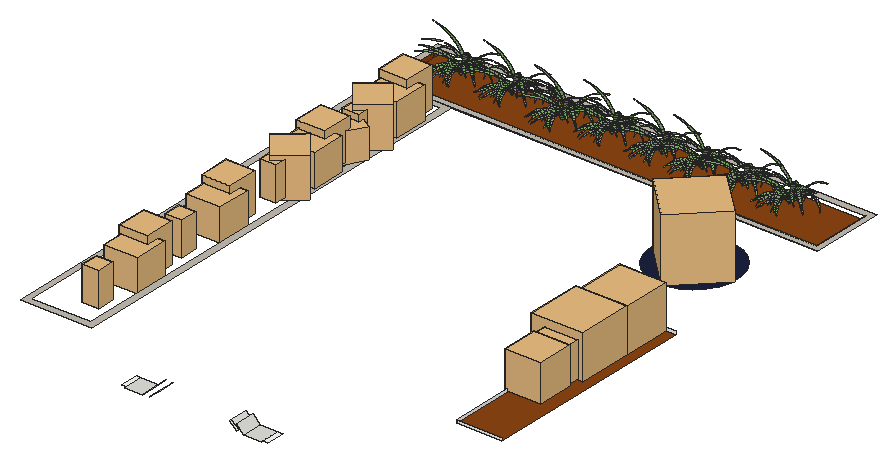
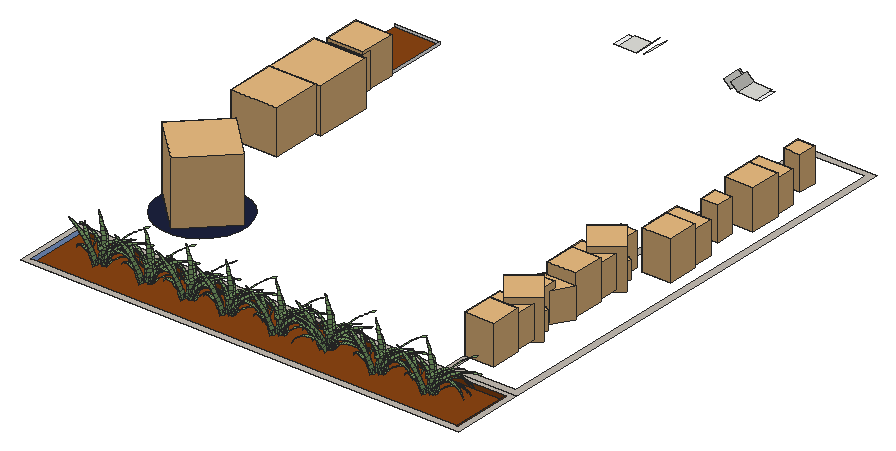
# SketchUp Ruby script. Lengths in inches.
U = 1.inch
M = Sketchup.active_model
def pt(a) = Geom::Point3d.new(a.map { |v| v * U })
def face(e, loops, mat)
  f = e.add_face(loops[0].map { |a| pt(a) })
  loops[1..].each { |l| e.add_face(l.map { |a| pt(a) }).erase! }
  f.material = f.back_material = mat if mat
  f
end
# faces: each face lists its corners as indices into pts; further lists are holes
def faces(e, pts, list, mat = nil) = list.each { |f| face(e, (f[0].is_a?(Array) ? f : [f]).map { |l| l.map { |i| pts[i] } }, mat) }
# xy, xz, yz: faces in a plane at the given z, y or x. An outline is a flat list of corners, or four numbers for a rectangle; further outlines are holes
def ring(l) = l.size == 4 ? [[l[0], l[1]], [l[2], l[1]], [l[2], l[3]], [l[0], l[3]]] : l.each_slice(2).to_a
def flat(e, list, mat, &to3) = list.each { |f| face(e, (f[0].is_a?(Array) ? f : [f]).map { |l| ring(l).map { |u, v| to3.(u, v) } }, mat) }
def xy(e, z, list, mat = nil) = flat(e, list, mat) { |x, y| [x, y, z] }
def xz(e, y, list, mat = nil) = flat(e, list, mat) { |x, z| [x, y, z] }
def yz(e, x, list, mat = nil) = flat(e, list, mat) { |y, z| [x, y, z] }
def lines(e, pts, list) = list.each { |a, b| e.add_line(pt(pts[a]), pt(pts[b])) }
# prism: a flat outline (further loops are holes) pulled along v
def prism(e, loops, v, mat = nil)
  f = face(e, loops, mat); d = Geom::Vector3d.new(v.map { |x| x * U })
  f.pushpull(f.normal.samedirection?(d) ? d.length : -d.length)
end
def box(e, o, s, mat = nil) = prism(e, [[o, [o[0] + s[0], o[1], o[2]], [o[0] + s[0], o[1] + s[1], o[2]], [o[0], o[1] + s[1], o[2]]]], [0, 0, s[2]], mat)
def at(x, y, z, deg = 0) = Geom::Transformation.translation(pt([x, y, z])) * Geom::Transformation.rotation(ORIGIN, Z_AXIS, deg.degrees)
def axes(o, x, y, z) = Geom::Transformation.new([*x, 0, *y, 0, *z, 0, *pt(o).to_a, 1])
def part(name) = M.definitions.add(name)
# library, detail: a bought-in or finely detailed component or shape, given as its bounding box
def library(name, o, s) = part(name).tap { |d| box(d.entities, o, s) }
def detail(e, o, s) = box(e.add_group.entities, o, s)
def put(e, d, t, mat = nil) = e.add_instance(d, t).tap { |i| i.material = mat if mat }
def group(e, t, mat = nil) = e.add_group.tap { |g| g.transformation = t; g.material = mat if mat }.entities
root = M.entities
M.materials.add("[0043_SaddleBrown]").color = [139, 69, 19]
M.materials.add("[0119_RosyBrown]").color = [29, 34, 63]
M.materials.add("[Color L01]").color = [158, 192, 255]
M.materials.add("[Color M00]").color = [255, 255, 255]
M.materials.add("[Field Rectangle Tile]").color = [196, 189, 179]
M.materials.add("dianella").color = [131, 171, 111]
c1 = library("Group38\#2",[14.01,28.44,-23.43],[18.58,18.32,38.89])
c2 = library("Group20\#1",[-20.81,-17.08,3.79],[39.86,39.43,37.51])
c3 = library("Group\#130",[-7.34,-1.2,0],[38.67,35.81,49.04])
c4 = library("Group\#339",[-7.85,-8.32,-6.76],[58.34,57.85,58.74])
c5 = library("Group\#332",[-8.56,-8.18,-3.7],[55.71,56.19,59.24])
c6 = library("Group\#329",[-12.44,-11,-10.61],[94.39,87.27,76.58])
c7 = library("Group\#292",[-21.05,-15.88,-13.81],[107.65,102.98,97.72])
c8 = library("Group\#74",[-84.69,-90.07,-0.36],[176.51,175.13,171.4])
c9 = library("Areca palm plant",[0,0,0],[49.1,36.6,54.46])
c10 = library("Water tank",[0,0,0],[57.22,57.22,62.99])
c11 = part("Shape Bender Component\#4")
p = [[0.27,1.78,0.46],[1.95,1.8,3.35],[1.95,4.67,3.35],[0.27,4.68,0.46],[3.06,1.81,4.8],[3.875,1.84,5.87],
  [3.875,4.64,5.87],[3.06,4.66,4.8],[6,1.9,8],[6,4.58,8],[27.35,3.23,6.09],[25.57,3.4375,7.9],
  [25.57,3.03,7.9],[23.28,2.8,9.61],[23.28,3.67,9.61],[7.08,1.93,8.8],[8.3,1.99,9.69],[8.3,4.5,9.69],
  [7.08,4.55,8.8],[23.04,2.78,9.74],[23.04,3.69,9.74],[20.86,3.86,10.86],[20.86,2.625,10.86],[10.73,2.08,10.92],
  [10.73,4.41,10.92],[12.13,2.13,11.33],[13.24,2.19,11.66],[13.24,4.3,11.66],[12.13,4.36,11.33],[18.35,2.46,11.63],
  [18.35,4.03,11.63],[15.79,2.32,11.89],[17.75,2.42,11.69],[17.75,4.07,11.69],[15.79,4.17,11.89]]
faces(c11.entities,p,[[0,1,2,3],[1,4,5,6,7,2],[5,8,9,6],[10,11,12],[13,12,11,14],[15,16,17,18,9,8],[19,13,14,20,21,22],[16,23,24,17],
  [23,25,26,27,28,24],[29,22,21,30],[31,32,29,30,33,34],[26,31,34,27]],"dianella")
c12 = part("Shape Bender Component\#7")
p = [[0.01,0.94,1.17],[0.04,0.96,6.32],[0.04,4.67,6.32],[0.01,4.68,1.17],[0.42,0.98,10.52],[0.51,1,11.45],
  [0.51,4.64,11.45],[0.42,4.66,10.52],[1.4,1.07,16.52],[1.4,4.57,16.52],[2.48,1.13,20.62],[2.71,1.16,21.49],
  [2.71,4.49,21.49],[2.48,4.52,20.625],[4.4375,1.21,26.32],[4.4375,4.46,26.32],[6.56,1.22,30.98],[6.56,4.47,30.98],
  [9.06,1.29,35.43],[9.06,4.38,35.43],[11.92,1.42,39.64],[11.92,4.23,39.64],[15.13,1.74,43.57],[15.13,4,43.57],
  [18.65,2.08,47.2],[18.65,3.67,47.2],[22.46,2.47,50.5],[22.46,3.14,50.5],[25.84,2.81,52.95]]
faces(c12.entities,p,[[0,1,2,3],[1,4,5,6,7,2],[5,8,9,6],[10,11,12,13,9,8],[11,14,15,12],[14,16,17,15],[16,18,19,17],[18,20,21,19],
  [20,22,23,21],[22,24,25,23],[24,26,27,25],[28,27,26]],"dianella")
c13 = part("Shape Bender Component\#5")
p = [[0.17,0.01,0.72],[1.09,0.03,4.5625],[1.09,3.73,4.5625],[0.17,3.75,0.72],[2.23,0.05,7.59],[2.48,0.0625,8.26],
  [2.48,3.71,8.26],[2.23,3.72,7.59],[4.33,0.14,11.74],[4.33,3.64,11.74],[6.2,0.2,14.41],[6.6,0.22,14.97],
  [6.6,3.56,14.97],[6.2,3.58,14.41],[9.26,0.35,17.88],[9.26,3.43,17.88],[12.27,0.4,20.43],[12.27,3.38,20.43],
  [15.58,0.51,22.59],[15.58,3.27,22.59],[19.13,0.73,24.3],[19.13,3.14,24.3],[22.875,1.08,25.56],[22.875,2.85,25.56],
  [26.75,1.47,26.33],[26.75,2.49,26.33],[30.68,1.86,26.6],[30.68,2.125,26.6],[33.95,1.875,26.45]]
faces(c13.entities,p,[[0,1,2,3],[1,4,5,6,7,2],[5,8,9,6],[8,10,11,12,13,9],[11,14,15,12],[14,16,17,15],[16,18,19,17],[18,20,21,19],
  [20,22,23,21],[22,24,25,23],[24,26,27,25],[28,27,26]],"dianella")
xy(root,281.8125,[[30,509.79,450,570]],"[0043_SaddleBrown]")
xy(root,285.0625,[[172.5,4,190.5,24],[289.5,4,307.5,24]])
xy(root,285.0625,[[168,6,172.5,24],[307.5,6,312,24]],"[Color M00]")
xy(root,286.25,[[398.2,388.3,408.88,390.95,418.5,396.27,426.42,403.9,432.1,413.32,435.14,423.88,435.35,434.88,432.7,445.55,427.38,455.18,419.75,463.1,410.34,468.77,399.77,471.82,388.77,472.02,378.1,469.375,368.47,464.06,360.55,456.43,354.88,447.01,351.83,436.44,351.63,425.45,354.27,414.77,359.59,405.15,367.22,397.23,376.64,391.55,387.21,388.51]],"[0119_RosyBrown]")
xy(root,286.25,[[[24,60.88,94.68,503.79],[30,66.88,88.68,497.79]],[[24,503.79,456,576],[30,509.79,450,570]]],"[Field Rectangle Tile]")
xy(root,289.375,[[411,114.58,456,328.96]],"[0043_SaddleBrown]")
xz(root,114.58,[[411,289.375,456,292.1875]],"[Color M00]")
xz(root,328.96,[[411,289.375,456,292.1875]],"[Color M00]")
xz(root,509.79,[[30,281.8125,94.68,286.25],[94.68,281.8125,350.9,286.25],[350.9,281.8125,410.59,286.25],[410.59,281.8125,450,286.25]],"[0043_SaddleBrown]")
yz(root,30,[[509.79,281.8125,570,286.25]],"[0043_SaddleBrown]")
yz(root,411,[[114.58,289.375,328.96,292.1875]],"[Color M00]")
yz(root,450,[[509.79,281.8125,570,286.25]],"[Color L01]")
p = [[190.5,24,285.0625],[190.5,4,285.0625],[196.91,4,292.04],[196.91,24,292.04],[283.09,24,292.04],[283.09,4,292.04],
  [289.5,4,285.0625],[289.5,24,285.0625],[196.93,6,286.04],[204.32,6,291.98],[204.32,4,291.98],[196.93,4,286.04],
  [275.8,6,291.98],[283.2,6,286.04],[283.2,4,286.04],[275.8,4,291.98],[196.93,24,286.04],[204.32,24,291.98],
  [275.8,24,291.98],[283.2,24,286.04]]
faces(root,p,[[0,1,2,3],[4,5,6,7],[8,9,10,11],[12,13,14,15],[9,8,16,17],[13,12,18,19]])
put(root,c1,axes([46.13,67.14,301.625],[0.8848,0,0],[0,0.94674,0],[0,0,0.85826]))
put(root,c2,axes([69.2,148.27,278.23],[0,0.85,0],[-0.85,0,0],[0,0,0.85]))
put(root,c3,axes([75.17,158.2,281.45],[0,0.79,0],[-0.79,0,0],[0,0,0.79]))
put(root,c4,axes([439.2,181.99,294.74],[0,0.616,0],[-0.616,0,0],[0,0,0.616]))
put(root,c1,axes([46.13,168.95,301.625],[0.8848,0,0],[0,0.94674,0],[0,0,0.85826]))
put(root,c5,axes([436.17,209.26,292.1875],[0,0.58004,0],[-0.58004,0,0],[0,0,0.58004]))
put(root,c2,axes([69.2,250.08,278.23],[0,0.85,0],[-0.85,0,0],[0,0,0.85]))
put(root,c6,axes([439.55,233.71,293.78],[0,0.58004,0],[-0.58004,0,0],[0,0,0.58004]))
put(root,c3,axes([75.17,260.02,281.45],[0,0.79,0],[-0.79,0,0],[0,0,0.79]))
put(root,c1,axes([59.43,268.9,310.82],[0.8848,0,0],[0,0.94674,0],[0,0,0.85826]))
put(root,c7,axes([439.1,290.93,294.59],[0,0.44269,0],[-0.44269,0,0],[0,0,0.44269]))
put(root,c8,axes([78.46,314.11,288.7],[-0.04961,-0.08593,0],[0.08593,-0.04961,0],[0,0,0.10522]))
put(root,c9,axes([57.34,326.66,288.73],[0.45017,-0.56191,0],[0.66137,0.52986,0],[0,0,0.72]))
put(root,c8,axes([78.46,341.36,288.7],[-0.04961,-0.08593,0],[0.08593,-0.04961,0],[0,0,0.10522]))
put(root,c2,axes([82.5,350.03,287.42],[0,0.85,0],[-0.85,0,0],[0,0,0.85]))
put(root,c8,axes([78.46,361.43,288.7],[-0.04961,-0.08593,0],[0.08593,-0.04961,0],[0,0,0.10522]))
put(root,c3,axes([88.47,359.97,290.64],[0,0.79,0],[-0.79,0,0],[0,0,0.79]))
put(root,c8,axes([80.72,391.29,288.72],[-0.08133,-0.14087,0],[0.14087,-0.08133,0],[0,0,0.1725]))
put(root,c1,axes([59.43,370.72,310.82],[0.8848,0,0],[0,0.94674,0],[0,0,0.85826]))
put(root,c8,axes([78.46,415.93,288.7],[-0.04961,-0.08593,0],[0.08593,-0.04961,0],[0,0,0.10522]))
put(root,c9,axes([57.34,428.47,288.73],[0.45017,-0.56191,0],[0.66137,0.52986,0],[0,0,0.72]))
put(root,c10,at(395.83,385.39,286.25,45))
put(root,c8,axes([78.46,443.18,288.7],[-0.04961,-0.08593,0],[0.08593,-0.04961,0],[0,0,0.10522]))
put(root,c2,axes([82.5,451.85,287.42],[0,0.85,0],[-0.85,0,0],[0,0,0.85]))
put(root,c8,axes([78.46,463.24,288.7],[-0.04961,-0.08593,0],[0.08593,-0.04961,0],[0,0,0.10522]))
put(root,c3,axes([88.47,461.78,290.64],[0,0.79,0],[-0.79,0,0],[0,0,0.79]))
put(root,c11,axes([179.97,534.78,303.24],[0.24384,-0.52892,-0.4943],[-0.96778,-0.07931,-0.14256],[-0.0628,-0.83154,0.27772]))
put(root,c11,axes([181.1,538.37,290.98],[0.29817,-0.958,-0.07367],[-0.95106,-0.29183,-0.10772],[-0.07571,-0.06137,0.93269]))
put(root,c11,axes([177.34,535.38,292.46],[-0.80902,-0.55509,-0.2049],[-0.50904,0.51531,0.6897],[0.29389,-0.63549,0.63055]))
put(root,c11,axes([179.04,537.68,296.61],[-0.6497,-0.66955,-0.47553],[-0.70108,0.35409,0.77459],[0.29389,-0.63549,0.79655]))
put(root,c12,axes([177.625,537.24,288.47],[-0.80902,-0.55509,-0.2049],[-0.58779,0.76402,0.28202],[0,-0.21952,0.66819]))
put(root,c11,axes([125.48,540.78,303.24],[0.24384,-0.52892,-0.4943],[-0.96778,-0.07931,-0.14256],[-0.0628,-0.83154,0.27772]))
put(root,c11,axes([223.89,540.78,303.24],[0.24384,-0.52892,-0.4943],[-0.96778,-0.07931,-0.14256],[-0.0628,-0.83154,0.27772]))
put(root,c11,axes([312.36,540.78,303.24],[0.24384,-0.52892,-0.4943],[-0.96778,-0.07931,-0.14256],[-0.0628,-0.83154,0.27772]))
put(root,c11,axes([398.57,540.78,303.24],[0.24384,-0.52892,-0.4943],[-0.96778,-0.07931,-0.14256],[-0.0628,-0.83154,0.27772]))
put(root,c11,axes([74.96,540.78,303.24],[0.24384,-0.52892,-0.4943],[-0.96778,-0.07931,-0.14256],[-0.0628,-0.83154,0.27772]))
put(root,c11,axes([273.45,540.78,303.24],[0.24384,-0.52892,-0.4943],[-0.96778,-0.07931,-0.14256],[-0.0628,-0.83154,0.27772]))
put(root,c11,axes([353.46,540.78,303.24],[0.24384,-0.52892,-0.4943],[-0.96778,-0.07931,-0.14256],[-0.0628,-0.83154,0.27772]))
put(root,c11,axes([179.17,538.82,288.84],[-0.07321,-0.77652,-0.15951],[-0.98564,0.05292,0.13125],[0.15553,-0.00912,0.89892]))
put(root,c13,axes([177.44,544.51,290.85],[0.73728,-0.63801,-0.23551],[-0.67559,-0.69627,-0.25701],[0,-0.29269,0.89092]))
put(root,c11,axes([178.21,540.91,291.93],[-0.6497,-0.66955,-0.37643],[-0.70108,0.35409,0.61317],[0.29389,-0.63549,0.63055]))
put(root,c11,axes([179.09,542.53,289.11],[-0.15013,-1.00719,0.03173],[-0.93144,0.16994,0.33137],[0.32821,0.01861,0.90518]))
put(root,c11,axes([183.75,543.31,304.24],[-0.1251,-0.86028,-0.44795],[-0.93281,0.27107,-0.22947],[-0.33797,-0.42973,0.79917]))
put(root,c11,axes([126.61,544.37,290.98],[0.29817,-0.958,-0.07367],[-0.95106,-0.29183,-0.10772],[-0.07571,-0.06137,0.93269]))
put(root,c11,axes([225.02,544.37,290.98],[0.29817,-0.958,-0.07367],[-0.95106,-0.29183,-0.10772],[-0.07571,-0.06137,0.93269]))
put(root,c11,axes([313.5,544.37,290.98],[0.29817,-0.958,-0.07367],[-0.95106,-0.29183,-0.10772],[-0.07571,-0.06137,0.93269]))
put(root,c11,axes([399.7,544.37,290.98],[0.29817,-0.958,-0.07367],[-0.95106,-0.29183,-0.10772],[-0.07571,-0.06137,0.93269]))
put(root,c11,axes([76.09,544.37,290.98],[0.29817,-0.958,-0.07367],[-0.95106,-0.29183,-0.10772],[-0.07571,-0.06137,0.93269]))
put(root,c11,axes([274.58,544.37,290.98],[0.29817,-0.958,-0.07367],[-0.95106,-0.29183,-0.10772],[-0.07571,-0.06137,0.93269]))
put(root,c11,axes([354.59,544.37,290.98],[0.29817,-0.958,-0.07367],[-0.95106,-0.29183,-0.10772],[-0.07571,-0.06137,0.93269]))
put(root,c13,axes([177.01,540.96,289.54],[-0.87036,-0.46503,-0.17166],[-0.49242,0.82194,0.3034],[0,-0.29269,0.89092]))
put(root,c11,axes([122.85,541.38,292.46],[-0.80902,-0.55509,-0.2049],[-0.50904,0.51531,0.6897],[0.29389,-0.63549,0.63055]))
put(root,c11,axes([221.26,541.38,292.46],[-0.80902,-0.55509,-0.2049],[-0.50904,0.51531,0.6897],[0.29389,-0.63549,0.63055]))
put(root,c11,axes([309.73,541.38,292.46],[-0.80902,-0.55509,-0.2049],[-0.50904,0.51531,0.6897],[0.29389,-0.63549,0.63055]))
put(root,c11,axes([395.9375,541.38,292.46],[-0.80902,-0.55509,-0.2049],[-0.50904,0.51531,0.6897],[0.29389,-0.63549,0.63055]))
put(root,c11,axes([72.33,541.38,292.46],[-0.80902,-0.55509,-0.2049],[-0.50904,0.51531,0.6897],[0.29389,-0.63549,0.63055]))
put(root,c11,axes([270.82,541.38,292.46],[-0.80902,-0.55509,-0.2049],[-0.50904,0.51531,0.6897],[0.29389,-0.63549,0.63055]))
put(root,c11,axes([350.83,541.38,292.46],[-0.80902,-0.55509,-0.2049],[-0.50904,0.51531,0.6897],[0.29389,-0.63549,0.63055]))
put(root,c11,axes([124.56,543.68,296.61],[-0.6497,-0.66955,-0.47553],[-0.70108,0.35409,0.77459],[0.29389,-0.63549,0.79655]))
put(root,c11,axes([222.96,543.68,296.61],[-0.6497,-0.66955,-0.47553],[-0.70108,0.35409,0.77459],[0.29389,-0.63549,0.79655]))
put(root,c11,axes([311.4375,543.68,296.61],[-0.6497,-0.66955,-0.47553],[-0.70108,0.35409,0.77459],[0.29389,-0.63549,0.79655]))
put(root,c11,axes([397.64,543.68,296.61],[-0.6497,-0.66955,-0.47553],[-0.70108,0.35409,0.77459],[0.29389,-0.63549,0.79655]))
put(root,c11,axes([74.04,543.68,296.61],[-0.6497,-0.66955,-0.47553],[-0.70108,0.35409,0.77459],[0.29389,-0.63549,0.79655]))
put(root,c11,axes([272.52,543.68,296.61],[-0.6497,-0.66955,-0.47553],[-0.70108,0.35409,0.77459],[0.29389,-0.63549,0.79655]))
put(root,c11,axes([352.53,543.68,296.61],[-0.6497,-0.66955,-0.47553],[-0.70108,0.35409,0.77459],[0.29389,-0.63549,0.79655]))
put(root,c11,axes([176.8125,539.01,288.83],[-0.80902,-0.55509,-0.2049],[-0.58779,0.76402,0.28202],[0,-0.29269,0.89092]))
put(root,c12,axes([178.66,546.14,291.6],[0.80902,-0.55509,-0.2049],[-0.58572,-0.78583,-0.20648],[0.03689,-0.1708,0.68355]))
put(root,c12,axes([123.14,543.24,288.47],[-0.80902,-0.55509,-0.2049],[-0.58779,0.76402,0.28202],[0,-0.21952,0.66819]))
put(root,c12,axes([221.54,543.24,288.47],[-0.80902,-0.55509,-0.2049],[-0.58779,0.76402,0.28202],[0,-0.21952,0.66819]))
put(root,c12,axes([310.02,543.24,288.47],[-0.80902,-0.55509,-0.2049],[-0.58779,0.76402,0.28202],[0,-0.21952,0.66819]))
put(root,c12,axes([396.23,543.24,288.47],[-0.80902,-0.55509,-0.2049],[-0.58779,0.76402,0.28202],[0,-0.21952,0.66819]))
put(root,c12,axes([72.62,543.24,288.47],[-0.80902,-0.55509,-0.2049],[-0.58779,0.76402,0.28202],[0,-0.21952,0.66819]))
put(root,c12,axes([271.1,543.24,288.47],[-0.80902,-0.55509,-0.2049],[-0.58779,0.76402,0.28202],[0,-0.21952,0.66819]))
put(root,c12,axes([351.11,543.24,288.47],[-0.80902,-0.55509,-0.2049],[-0.58779,0.76402,0.28202],[0,-0.21952,0.66819]))
put(root,c11,axes([183.29,544.95,303.29],[0.62783,-0.50605,-0.54777],[-0.69981,-0.69909,-0.12156],[0.34071,-0.50341,0.75971]))
put(root,c11,axes([182.25,545.58,291.4375],[0.77059,-0.63454,0.09042],[-0.58779,-0.76402,-0.28202],[-0.23015,-0.11943,0.90121]))
put(root,c11,axes([124.68,544.82,288.84],[-0.07321,-0.77652,-0.15951],[-0.98564,0.05292,0.13125],[0.15553,-0.00912,0.89892]))
put(root,c11,axes([223.09,544.82,288.84],[-0.07321,-0.77652,-0.15951],[-0.98564,0.05292,0.13125],[0.15553,-0.00912,0.89892]))
put(root,c11,axes([311.57,544.82,288.84],[-0.07321,-0.77652,-0.15951],[-0.98564,0.05292,0.13125],[0.15553,-0.00912,0.89892]))
put(root,c11,axes([397.77,544.82,288.84],[-0.07321,-0.77652,-0.15951],[-0.98564,0.05292,0.13125],[0.15553,-0.00912,0.89892]))
put(root,c11,axes([74.16,544.82,288.84],[-0.07321,-0.77652,-0.15951],[-0.98564,0.05292,0.13125],[0.15553,-0.00912,0.89892]))
put(root,c11,axes([272.65,544.82,288.84],[-0.07321,-0.77652,-0.15951],[-0.98564,0.05292,0.13125],[0.15553,-0.00912,0.89892]))
put(root,c11,axes([352.66,544.82,288.84],[-0.07321,-0.77652,-0.15951],[-0.98564,0.05292,0.13125],[0.15553,-0.00912,0.89892]))
put(root,c13,axes([122.96,550.51,290.85],[0.73728,-0.63801,-0.23551],[-0.67559,-0.69627,-0.25701],[0,-0.29269,0.89092]))
put(root,c13,axes([221.36,550.51,290.85],[0.73728,-0.63801,-0.23551],[-0.67559,-0.69627,-0.25701],[0,-0.29269,0.89092]))
put(root,c13,axes([309.84,550.51,290.85],[0.73728,-0.63801,-0.23551],[-0.67559,-0.69627,-0.25701],[0,-0.29269,0.89092]))
put(root,c13,axes([396.04,550.51,290.85],[0.73728,-0.63801,-0.23551],[-0.67559,-0.69627,-0.25701],[0,-0.29269,0.89092]))
put(root,c13,axes([72.4375,550.51,290.85],[0.73728,-0.63801,-0.23551],[-0.67559,-0.69627,-0.25701],[0,-0.29269,0.89092]))
put(root,c13,axes([270.92,550.51,290.85],[0.73728,-0.63801,-0.23551],[-0.67559,-0.69627,-0.25701],[0,-0.29269,0.89092]))
put(root,c13,axes([350.93,550.51,290.85],[0.73728,-0.63801,-0.23551],[-0.67559,-0.69627,-0.25701],[0,-0.29269,0.89092]))
put(root,c11,axes([123.73,546.91,291.93],[-0.6497,-0.66955,-0.37643],[-0.70108,0.35409,0.61317],[0.29389,-0.63549,0.63055]))
put(root,c11,axes([222.13,546.91,291.93],[-0.6497,-0.66955,-0.37643],[-0.70108,0.35409,0.61317],[0.29389,-0.63549,0.63055]))
put(root,c11,axes([310.61,546.91,291.93],[-0.6497,-0.66955,-0.37643],[-0.70108,0.35409,0.61317],[0.29389,-0.63549,0.63055]))
put(root,c11,axes([396.81,546.91,291.93],[-0.6497,-0.66955,-0.37643],[-0.70108,0.35409,0.61317],[0.29389,-0.63549,0.63055]))
put(root,c11,axes([73.21,546.91,291.93],[-0.6497,-0.66955,-0.37643],[-0.70108,0.35409,0.61317],[0.29389,-0.63549,0.63055]))
put(root,c11,axes([271.69,546.91,291.93],[-0.6497,-0.66955,-0.37643],[-0.70108,0.35409,0.61317],[0.29389,-0.63549,0.63055]))
put(root,c11,axes([351.7,546.91,291.93],[-0.6497,-0.66955,-0.37643],[-0.70108,0.35409,0.61317],[0.29389,-0.63549,0.63055]))
put(root,c11,axes([124.61,548.53,289.11],[-0.15013,-1.00719,0.03173],[-0.93144,0.16994,0.33137],[0.32821,0.01861,0.90518]))
put(root,c11,axes([223.01,548.53,289.11],[-0.15013,-1.00719,0.03173],[-0.93144,0.16994,0.33137],[0.32821,0.01861,0.90518]))
put(root,c11,axes([311.49,548.53,289.11],[-0.15013,-1.00719,0.03173],[-0.93144,0.16994,0.33137],[0.32821,0.01861,0.90518]))
put(root,c11,axes([397.69,548.53,289.11],[-0.15013,-1.00719,0.03173],[-0.93144,0.16994,0.33137],[0.32821,0.01861,0.90518]))
put(root,c11,axes([74.08,548.53,289.11],[-0.15013,-1.00719,0.03173],[-0.93144,0.16994,0.33137],[0.32821,0.01861,0.90518]))
put(root,c11,axes([272.57,548.53,289.11],[-0.15013,-1.00719,0.03173],[-0.93144,0.16994,0.33137],[0.32821,0.01861,0.90518]))
put(root,c11,axes([352.58,548.53,289.11],[-0.15013,-1.00719,0.03173],[-0.93144,0.16994,0.33137],[0.32821,0.01861,0.90518]))
put(root,c11,axes([129.27,549.31,304.24],[-0.1251,-0.86028,-0.44795],[-0.93281,0.27107,-0.22947],[-0.33797,-0.42973,0.79917]))
put(root,c11,axes([227.67,549.31,304.24],[-0.1251,-0.86028,-0.44795],[-0.93281,0.27107,-0.22947],[-0.33797,-0.42973,0.79917]))
put(root,c11,axes([316.15,549.31,304.24],[-0.1251,-0.86028,-0.44795],[-0.93281,0.27107,-0.22947],[-0.33797,-0.42973,0.79917]))
put(root,c11,axes([402.35,549.31,304.24],[-0.1251,-0.86028,-0.44795],[-0.93281,0.27107,-0.22947],[-0.33797,-0.42973,0.79917]))
put(root,c11,axes([78.75,549.31,304.24],[-0.1251,-0.86028,-0.44795],[-0.93281,0.27107,-0.22947],[-0.33797,-0.42973,0.79917]))
put(root,c11,axes([277.23,549.31,304.24],[-0.1251,-0.86028,-0.44795],[-0.93281,0.27107,-0.22947],[-0.33797,-0.42973,0.79917]))
put(root,c11,axes([357.24,549.31,304.24],[-0.1251,-0.86028,-0.44795],[-0.93281,0.27107,-0.22947],[-0.33797,-0.42973,0.79917]))
put(root,c13,axes([180.42,545.41,290.12],[0.64289,-0.76505,-0.03723],[0.71567,0.6173,-0.32675],[0.24294,0.16325,0.84049]))
put(root,c13,axes([179.18,542.62,291.85],[-0.77816,-0.62697,-0.04132],[-0.58344,0.74353,-0.3627],[-0.20696,0.20696,0.93295]))
put(root,c13,axes([122.53,546.96,289.54],[-0.87036,-0.46503,-0.17166],[-0.49242,0.82194,0.3034],[0,-0.29269,0.89092]))
put(root,c13,axes([220.93,546.96,289.54],[-0.87036,-0.46503,-0.17166],[-0.49242,0.82194,0.3034],[0,-0.29269,0.89092]))
put(root,c13,axes([309.41,546.96,289.54],[-0.87036,-0.46503,-0.17166],[-0.49242,0.82194,0.3034],[0,-0.29269,0.89092]))
put(root,c13,axes([395.61,546.96,289.54],[-0.87036,-0.46503,-0.17166],[-0.49242,0.82194,0.3034],[0,-0.29269,0.89092]))
put(root,c13,axes([72.01,546.96,289.54],[-0.87036,-0.46503,-0.17166],[-0.49242,0.82194,0.3034],[0,-0.29269,0.89092]))
put(root,c13,axes([270.49,546.96,289.54],[-0.87036,-0.46503,-0.17166],[-0.49242,0.82194,0.3034],[0,-0.29269,0.89092]))
put(root,c13,axes([350.5,546.96,289.54],[-0.87036,-0.46503,-0.17166],[-0.49242,0.82194,0.3034],[0,-0.29269,0.89092]))
put(root,c13,axes([176.125,545.07,291.0625],[0.99357,-0.10691,-0.03946],[-0.1132,-0.93831,-0.34636],[0,-0.29269,0.89092]))
put(root,c11,axes([122.33,545.01,288.83],[-0.80902,-0.55509,-0.2049],[-0.58779,0.76402,0.28202],[0,-0.29269,0.89092]))
put(root,c11,axes([220.73,545.01,288.83],[-0.80902,-0.55509,-0.2049],[-0.58779,0.76402,0.28202],[0,-0.29269,0.89092]))
put(root,c11,axes([309.21,545.01,288.83],[-0.80902,-0.55509,-0.2049],[-0.58779,0.76402,0.28202],[0,-0.29269,0.89092]))
put(root,c11,axes([395.41,545.01,288.83],[-0.80902,-0.55509,-0.2049],[-0.58779,0.76402,0.28202],[0,-0.29269,0.89092]))
put(root,c11,axes([71.81,545.01,288.83],[-0.80902,-0.55509,-0.2049],[-0.58779,0.76402,0.28202],[0,-0.29269,0.89092]))
put(root,c11,axes([270.29,545.01,288.83],[-0.80902,-0.55509,-0.2049],[-0.58779,0.76402,0.28202],[0,-0.29269,0.89092]))
put(root,c11,axes([350.3,545.01,288.83],[-0.80902,-0.55509,-0.2049],[-0.58779,0.76402,0.28202],[0,-0.29269,0.89092]))
put(root,c12,axes([124.18,552.14,291.6],[0.80902,-0.55509,-0.2049],[-0.58572,-0.78583,-0.20648],[0.03689,-0.1708,0.68355]))
put(root,c12,axes([222.58,552.14,291.6],[0.80902,-0.55509,-0.2049],[-0.58572,-0.78583,-0.20648],[0.03689,-0.1708,0.68355]))
put(root,c12,axes([311.06,552.14,291.6],[0.80902,-0.55509,-0.2049],[-0.58572,-0.78583,-0.20648],[0.03689,-0.1708,0.68355]))
put(root,c12,axes([397.26,552.14,291.6],[0.80902,-0.55509,-0.2049],[-0.58572,-0.78583,-0.20648],[0.03689,-0.1708,0.68355]))
put(root,c12,axes([73.66,552.14,291.6],[0.80902,-0.55509,-0.2049],[-0.58572,-0.78583,-0.20648],[0.03689,-0.1708,0.68355]))
put(root,c12,axes([272.14,552.14,291.6],[0.80902,-0.55509,-0.2049],[-0.58572,-0.78583,-0.20648],[0.03689,-0.1708,0.68355]))
put(root,c12,axes([352.15,552.14,291.6],[0.80902,-0.55509,-0.2049],[-0.58572,-0.78583,-0.20648],[0.03689,-0.1708,0.68355]))
put(root,c11,axes([128.81,550.95,303.29],[0.62783,-0.50605,-0.54777],[-0.69981,-0.69909,-0.12156],[0.34071,-0.50341,0.75971]))
put(root,c11,axes([227.21,550.95,303.29],[0.62783,-0.50605,-0.54777],[-0.69981,-0.69909,-0.12156],[0.34071,-0.50341,0.75971]))
put(root,c11,axes([315.6875,550.95,303.29],[0.62783,-0.50605,-0.54777],[-0.69981,-0.69909,-0.12156],[0.34071,-0.50341,0.75971]))
put(root,c11,axes([401.89,550.95,303.29],[0.62783,-0.50605,-0.54777],[-0.69981,-0.69909,-0.12156],[0.34071,-0.50341,0.75971]))
put(root,c11,axes([78.29,550.95,303.29],[0.62783,-0.50605,-0.54777],[-0.69981,-0.69909,-0.12156],[0.34071,-0.50341,0.75971]))
put(root,c11,axes([276.77,550.95,303.29],[0.62783,-0.50605,-0.54777],[-0.69981,-0.69909,-0.12156],[0.34071,-0.50341,0.75971]))
put(root,c11,axes([356.78,550.95,303.29],[0.62783,-0.50605,-0.54777],[-0.69981,-0.69909,-0.12156],[0.34071,-0.50341,0.75971]))
put(root,c11,axes([127.76,551.58,291.4375],[0.77059,-0.63454,0.09042],[-0.58779,-0.76402,-0.28202],[-0.23015,-0.11943,0.90121]))
put(root,c11,axes([226.17,551.58,291.4375],[0.77059,-0.63454,0.09042],[-0.58779,-0.76402,-0.28202],[-0.23015,-0.11943,0.90121]))
put(root,c11,axes([314.64,551.58,291.4375],[0.77059,-0.63454,0.09042],[-0.58779,-0.76402,-0.28202],[-0.23015,-0.11943,0.90121]))
put(root,c11,axes([400.85,551.58,291.4375],[0.77059,-0.63454,0.09042],[-0.58779,-0.76402,-0.28202],[-0.23015,-0.11943,0.90121]))
put(root,c11,axes([77.24,551.58,291.4375],[0.77059,-0.63454,0.09042],[-0.58779,-0.76402,-0.28202],[-0.23015,-0.11943,0.90121]))
put(root,c11,axes([275.73,551.58,291.4375],[0.77059,-0.63454,0.09042],[-0.58779,-0.76402,-0.28202],[-0.23015,-0.11943,0.90121]))
put(root,c11,axes([355.74,551.58,291.4375],[0.77059,-0.63454,0.09042],[-0.58779,-0.76402,-0.28202],[-0.23015,-0.11943,0.90121]))
put(root,c11,axes([174.03,537.64,304.66],[-0.80177,-0.08612,-0.57361],[0.00051,0.98917,-0.12729],[-0.59688,0.11504,0.79555]))
put(root,c11,axes([181.38,542.48,294.38],[0.91196,-0.3619,-0.1933],[0.30631,0.914,-0.26606],[0.24294,0.16325,0.84049]))
put(root,c13,axes([125.9375,551.41,290.12],[0.64289,-0.76505,-0.03723],[0.71567,0.6173,-0.32675],[0.24294,0.16325,0.84049]))
put(root,c13,axes([224.34,551.41,290.12],[0.64289,-0.76505,-0.03723],[0.71567,0.6173,-0.32675],[0.24294,0.16325,0.84049]))
put(root,c13,axes([312.82,551.41,290.12],[0.64289,-0.76505,-0.03723],[0.71567,0.6173,-0.32675],[0.24294,0.16325,0.84049]))
put(root,c13,axes([399.03,551.41,290.12],[0.64289,-0.76505,-0.03723],[0.71567,0.6173,-0.32675],[0.24294,0.16325,0.84049]))
put(root,c13,axes([75.42,551.41,290.12],[0.64289,-0.76505,-0.03723],[0.71567,0.6173,-0.32675],[0.24294,0.16325,0.84049]))
put(root,c13,axes([273.9,551.41,290.12],[0.64289,-0.76505,-0.03723],[0.71567,0.6173,-0.32675],[0.24294,0.16325,0.84049]))
put(root,c13,axes([353.91,551.41,290.12],[0.64289,-0.76505,-0.03723],[0.71567,0.6173,-0.32675],[0.24294,0.16325,0.84049]))
put(root,c13,axes([124.7,548.62,291.85],[-0.77816,-0.62697,-0.04132],[-0.58344,0.74353,-0.3627],[-0.20696,0.20696,0.93295]))
put(root,c13,axes([223.1,548.62,291.85],[-0.77816,-0.62697,-0.04132],[-0.58344,0.74353,-0.3627],[-0.20696,0.20696,0.93295]))
put(root,c13,axes([311.58,548.62,291.85],[-0.77816,-0.62697,-0.04132],[-0.58344,0.74353,-0.3627],[-0.20696,0.20696,0.93295]))
put(root,c13,axes([397.78,548.62,291.85],[-0.77816,-0.62697,-0.04132],[-0.58344,0.74353,-0.3627],[-0.20696,0.20696,0.93295]))
put(root,c13,axes([74.17,548.62,291.85],[-0.77816,-0.62697,-0.04132],[-0.58344,0.74353,-0.3627],[-0.20696,0.20696,0.93295]))
put(root,c13,axes([272.66,548.62,291.85],[-0.77816,-0.62697,-0.04132],[-0.58344,0.74353,-0.3627],[-0.20696,0.20696,0.93295]))
put(root,c13,axes([352.67,548.62,291.85],[-0.77816,-0.62697,-0.04132],[-0.58344,0.74353,-0.3627],[-0.20696,0.20696,0.93295]))
put(root,c12,axes([180.95,542.7,290.625],[0.91196,-0.3619,-0.1933],[0.32556,0.92445,-0.19479],[0.16234,0.06465,0.64486]))
put(root,c12,axes([178.14,540.07,292.41],[-0.96457,-0.17955,-0.21457],[-0.1415,0.96983,-0.21622],[-0.14686,0.09469,0.71579]))
put(root,c11,axes([171.15,541.22,296.58],[-0.96457,-0.17955,-0.21457],[-0.12461,0.95587,-0.29533],[-0.20696,0.20696,0.93295]))
put(root,c13,axes([121.64,551.07,291.0625],[0.99357,-0.10691,-0.03946],[-0.1132,-0.93831,-0.34636],[0,-0.29269,0.89092]))
put(root,c13,axes([220.05,551.07,291.0625],[0.99357,-0.10691,-0.03946],[-0.1132,-0.93831,-0.34636],[0,-0.29269,0.89092]))
put(root,c13,axes([308.52,551.07,291.0625],[0.99357,-0.10691,-0.03946],[-0.1132,-0.93831,-0.34636],[0,-0.29269,0.89092]))
put(root,c13,axes([394.73,551.07,291.0625],[0.99357,-0.10691,-0.03946],[-0.1132,-0.93831,-0.34636],[0,-0.29269,0.89092]))
put(root,c13,axes([71.12,551.07,291.0625],[0.99357,-0.10691,-0.03946],[-0.1132,-0.93831,-0.34636],[0,-0.29269,0.89092]))
put(root,c13,axes([269.61,551.07,291.0625],[0.99357,-0.10691,-0.03946],[-0.1132,-0.93831,-0.34636],[0,-0.29269,0.89092]))
put(root,c13,axes([349.62,551.07,291.0625],[0.99357,-0.10691,-0.03946],[-0.1132,-0.93831,-0.34636],[0,-0.29269,0.89092]))
put(root,c13,axes([177.18,544.63,289.92],[0.94077,-0.2561,-0.22218],[0.2011,0.94909,-0.24247],[0.24294,0.16325,0.84049]))
put(root,c13,axes([177.85,542.09,291.63],[-0.97248,-0.07019,-0.24662],[-0.01462,0.97005,-0.26914],[-0.20696,0.20696,0.93295]))
put(root,c11,axes([119.54,543.64,304.66],[-0.80177,-0.08612,-0.57361],[0.00051,0.98917,-0.12729],[-0.59688,0.11504,0.79555]))
put(root,c11,axes([217.95,543.64,304.66],[-0.80177,-0.08612,-0.57361],[0.00051,0.98917,-0.12729],[-0.59688,0.11504,0.79555]))
put(root,c11,axes([306.42,543.64,304.66],[-0.80177,-0.08612,-0.57361],[0.00051,0.98917,-0.12729],[-0.59688,0.11504,0.79555]))
put(root,c11,axes([392.63,543.64,304.66],[-0.80177,-0.08612,-0.57361],[0.00051,0.98917,-0.12729],[-0.59688,0.11504,0.79555]))
put(root,c11,axes([69.02,543.64,304.66],[-0.80177,-0.08612,-0.57361],[0.00051,0.98917,-0.12729],[-0.59688,0.11504,0.79555]))
put(root,c11,axes([267.51,543.64,304.66],[-0.80177,-0.08612,-0.57361],[0.00051,0.98917,-0.12729],[-0.59688,0.11504,0.79555]))
put(root,c11,axes([347.52,543.64,304.66],[-0.80177,-0.08612,-0.57361],[0.00051,0.98917,-0.12729],[-0.59688,0.11504,0.79555]))
put(root,c11,axes([126.9,548.48,294.38],[0.91196,-0.3619,-0.1933],[0.30631,0.914,-0.26606],[0.24294,0.16325,0.84049]))
put(root,c11,axes([225.3,548.48,294.38],[0.91196,-0.3619,-0.1933],[0.30631,0.914,-0.26606],[0.24294,0.16325,0.84049]))
put(root,c11,axes([313.78,548.48,294.38],[0.91196,-0.3619,-0.1933],[0.30631,0.914,-0.26606],[0.24294,0.16325,0.84049]))
put(root,c11,axes([399.98,548.48,294.38],[0.91196,-0.3619,-0.1933],[0.30631,0.914,-0.26606],[0.24294,0.16325,0.84049]))
put(root,c11,axes([76.38,548.48,294.38],[0.91196,-0.3619,-0.1933],[0.30631,0.914,-0.26606],[0.24294,0.16325,0.84049]))
put(root,c11,axes([274.86,548.48,294.38],[0.91196,-0.3619,-0.1933],[0.30631,0.914,-0.26606],[0.24294,0.16325,0.84049]))
put(root,c11,axes([354.875,548.48,294.38],[0.91196,-0.3619,-0.1933],[0.30631,0.914,-0.26606],[0.24294,0.16325,0.84049]))
put(root,c13,axes([181.27,540.74,291.2],[0.98276,0.1646,0.08419],[-0.14484,0.96332,-0.19265],[-0.10945,0.21065,0.86584]))
put(root,c12,axes([126.46,548.7,290.625],[0.91196,-0.3619,-0.1933],[0.32556,0.92445,-0.19479],[0.16234,0.06465,0.64486]))
put(root,c12,axes([224.87,548.7,290.625],[0.91196,-0.3619,-0.1933],[0.32556,0.92445,-0.19479],[0.16234,0.06465,0.64486]))
put(root,c12,axes([313.34,548.7,290.625],[0.91196,-0.3619,-0.1933],[0.32556,0.92445,-0.19479],[0.16234,0.06465,0.64486]))
put(root,c12,axes([399.55,548.7,290.625],[0.91196,-0.3619,-0.1933],[0.32556,0.92445,-0.19479],[0.16234,0.06465,0.64486]))
put(root,c12,axes([75.94,548.7,290.625],[0.91196,-0.3619,-0.1933],[0.32556,0.92445,-0.19479],[0.16234,0.06465,0.64486]))
put(root,c12,axes([274.43,548.7,290.625],[0.91196,-0.3619,-0.1933],[0.32556,0.92445,-0.19479],[0.16234,0.06465,0.64486]))
put(root,c12,axes([354.4375,548.7,290.625],[0.91196,-0.3619,-0.1933],[0.32556,0.92445,-0.19479],[0.16234,0.06465,0.64486]))
put(root,c11,axes([181.77,541.1,293.64],[0.91783,0.24445,-0.31277],[-0.28823,0.95215,-0.10163],[0.24294,0.16325,0.84049]))
put(root,c12,axes([123.66,546.07,292.41],[-0.96457,-0.17955,-0.21457],[-0.1415,0.96983,-0.21622],[-0.14686,0.09469,0.71579]))
put(root,c12,axes([222.07,546.07,292.41],[-0.96457,-0.17955,-0.21457],[-0.1415,0.96983,-0.21622],[-0.14686,0.09469,0.71579]))
put(root,c12,axes([310.54,546.07,292.41],[-0.96457,-0.17955,-0.21457],[-0.1415,0.96983,-0.21622],[-0.14686,0.09469,0.71579]))
put(root,c12,axes([396.75,546.07,292.41],[-0.96457,-0.17955,-0.21457],[-0.1415,0.96983,-0.21622],[-0.14686,0.09469,0.71579]))
put(root,c12,axes([73.14,546.07,292.41],[-0.96457,-0.17955,-0.21457],[-0.1415,0.96983,-0.21622],[-0.14686,0.09469,0.71579]))
put(root,c12,axes([271.625,546.07,292.41],[-0.96457,-0.17955,-0.21457],[-0.1415,0.96983,-0.21622],[-0.14686,0.09469,0.71579]))
